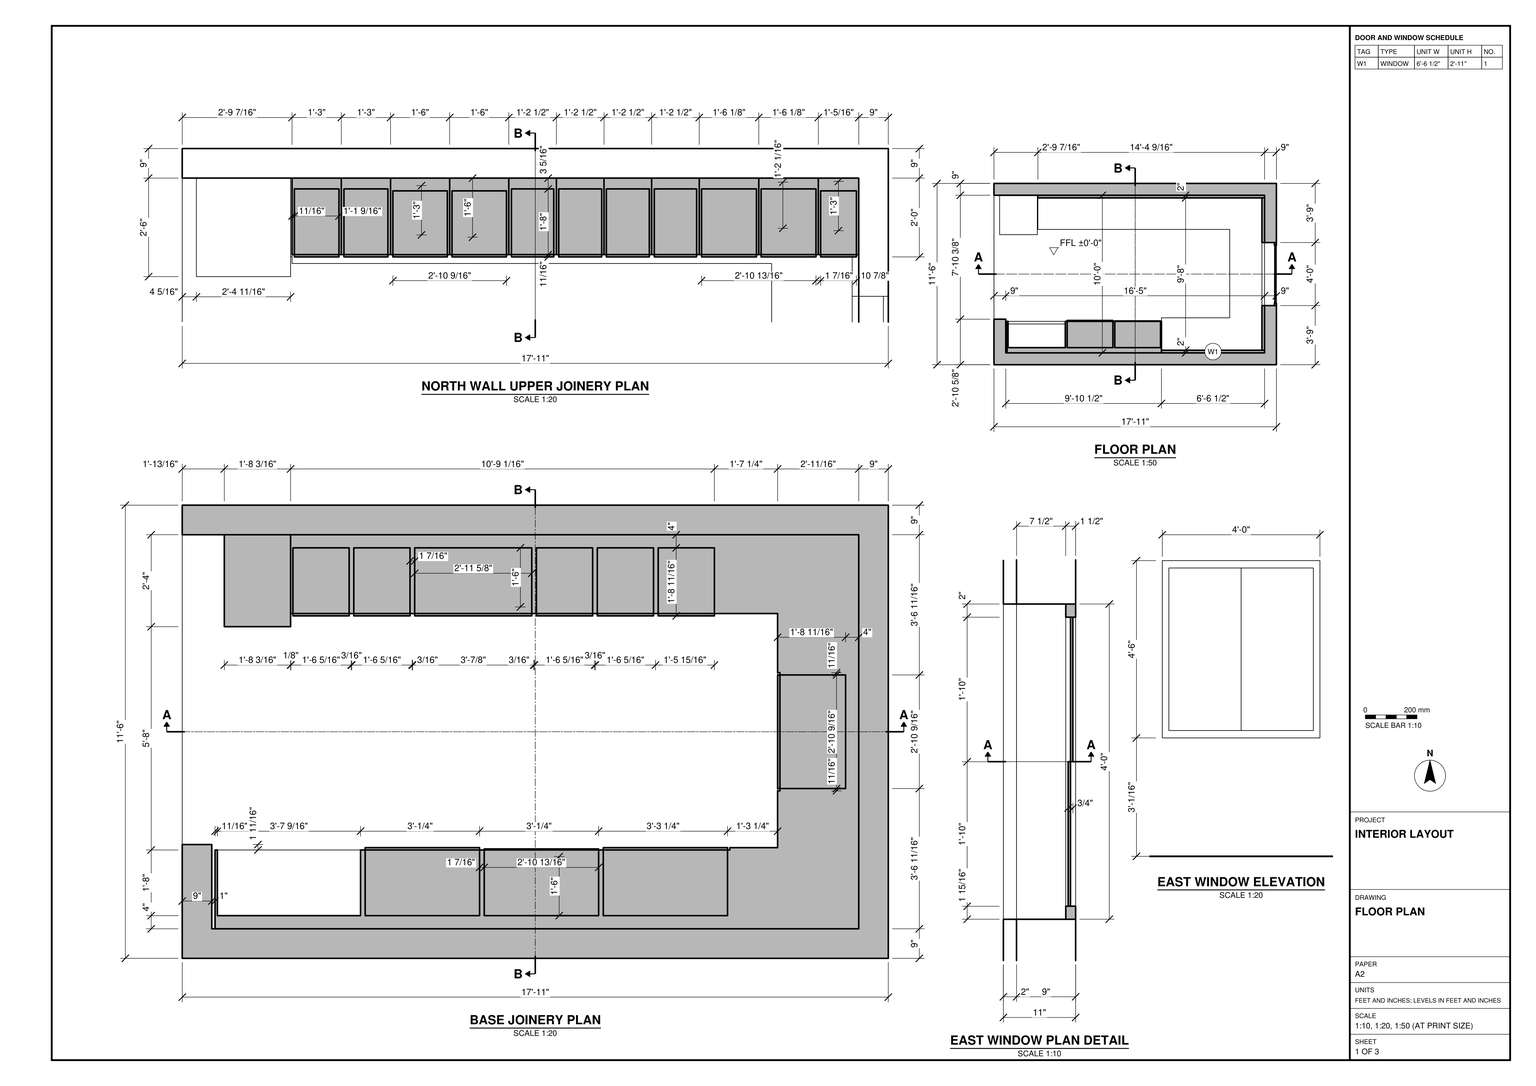
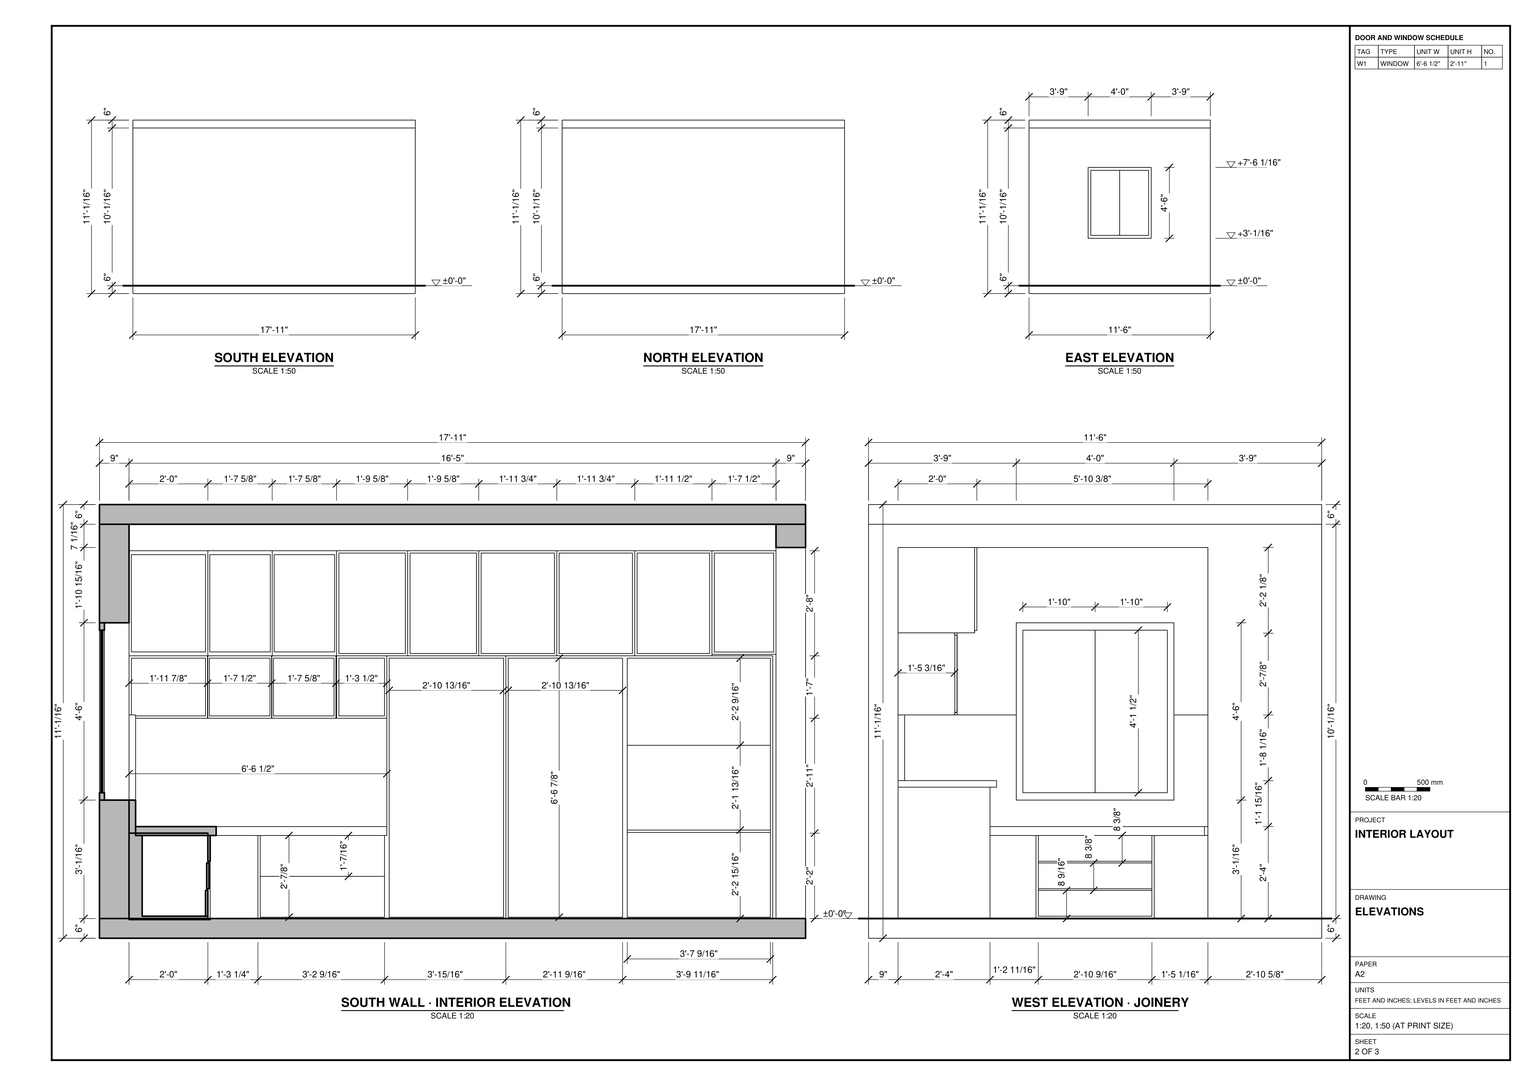
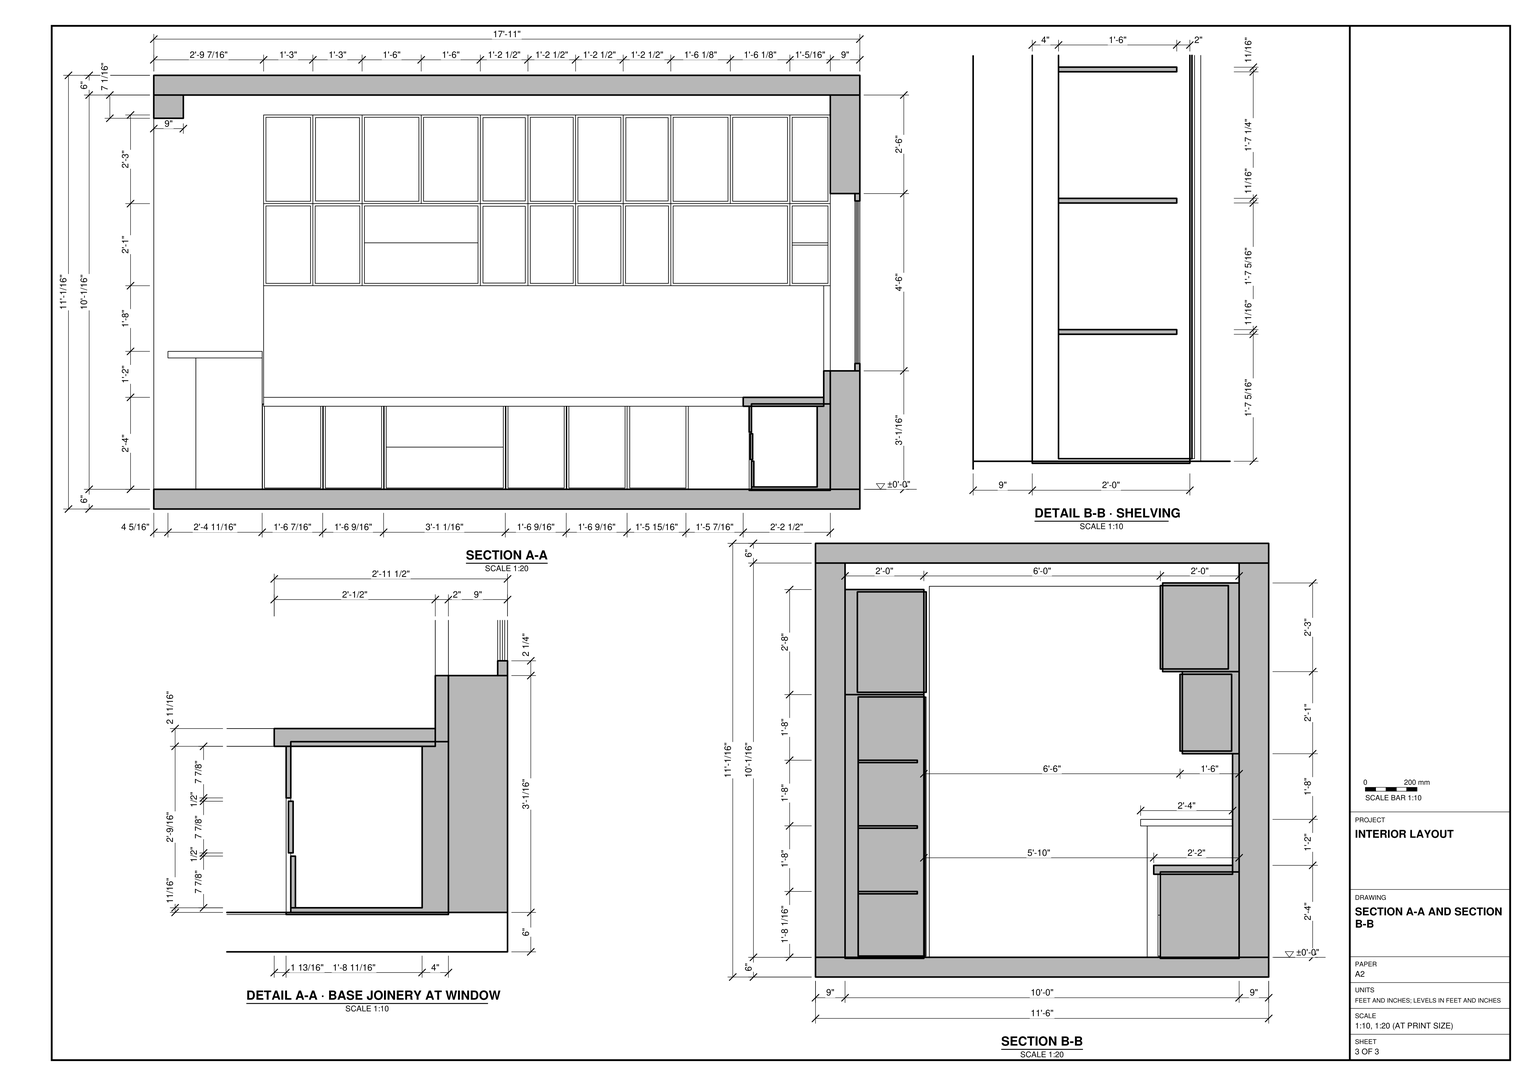
Build the room and its fitted joinery in SketchUp using task_files/diagram_01.pdf. Work in feet and inches. Set the finished floor level to ±0'-0". The overall shell measures 17'-11" east to west, 11'-6" north to south and 11'-1/16" high. Model the floor slab, top slab and walls at the thicknesses drawn, retaining the open portion of the west side shown in plan. Place the windows from the floor plan and use the east window detail for its frame and central division.

Use the base joinery plan to lay out the cabinets along the north and south walls and the connecting run beneath the east window. On the north wall, model the counter over the base units and the two tiers of upper cabinets. Use the sections to set the different cabinet depths. On the south wall, distinguish the low counter area, the tall storage bays and the stacked compartments beneath the continuous upper row. Include the drawer divisions below the east window and the internal shelving shown in detail.

Keep shell elements and individual joinery pieces in separate groups or components, and use components for repeated parts. Any decor or loose items may be suitable library components. Save one SketchUp model as output_files/fitted_storage_room_with_perimeter_cabinetry.skp.

# SketchUp Ruby script. Lengths in inches.
U = 1.inch
M = Sketchup.active_model
def pt(a) = Geom::Point3d.new(a.map { |v| v * U })
def face(e, loops, mat)
  f = e.add_face(loops[0].map { |a| pt(a) })
  loops[1..].each { |l| e.add_face(l.map { |a| pt(a) }).erase! }
  f.material = f.back_material = mat if mat
  f
end
# faces: each face lists its corners as indices into pts; further lists are holes
def faces(e, pts, list, mat = nil) = list.each { |f| face(e, (f[0].is_a?(Array) ? f : [f]).map { |l| l.map { |i| pts[i] } }, mat) }
# xy, xz, yz: faces in a plane at the given z, y or x. An outline is a flat list of corners, or four numbers for a rectangle; further outlines are holes
def ring(l) = l.size == 4 ? [[l[0], l[1]], [l[2], l[1]], [l[2], l[3]], [l[0], l[3]]] : l.each_slice(2).to_a
def flat(e, list, mat, &to3) = list.each { |f| face(e, (f[0].is_a?(Array) ? f : [f]).map { |l| ring(l).map { |u, v| to3.(u, v) } }, mat) }
def xy(e, z, list, mat = nil) = flat(e, list, mat) { |x, y| [x, y, z] }
def xz(e, y, list, mat = nil) = flat(e, list, mat) { |x, z| [x, y, z] }
def yz(e, x, list, mat = nil) = flat(e, list, mat) { |y, z| [x, y, z] }
def lines(e, pts, list) = list.each { |a, b| e.add_line(pt(pts[a]), pt(pts[b])) }
# prism: a flat outline (further loops are holes) pulled along v
def prism(e, loops, v, mat = nil)
  f = face(e, loops, mat); d = Geom::Vector3d.new(v.map { |x| x * U })
  f.pushpull(f.normal.samedirection?(d) ? d.length : -d.length)
end
def box(e, o, s, mat = nil) = prism(e, [[o, [o[0] + s[0], o[1], o[2]], [o[0] + s[0], o[1] + s[1], o[2]], [o[0], o[1] + s[1], o[2]]]], [0, 0, s[2]], mat)
def at(x, y, z, deg = 0) = Geom::Transformation.translation(pt([x, y, z])) * Geom::Transformation.rotation(ORIGIN, Z_AXIS, deg.degrees)
def axes(o, x, y, z) = Geom::Transformation.new([*x, 0, *y, 0, *z, 0, *pt(o).to_a, 1])
def part(name) = M.definitions.add(name)
# library, detail: a bought-in or finely detailed component or shape, given as its bounding box
def library(name, o, s) = part(name).tap { |d| box(d.entities, o, s) }
def detail(e, o, s) = box(e.add_group.entities, o, s)
def put(e, d, t, mat = nil) = e.add_instance(d, t).tap { |i| i.material = mat if mat }
def group(e, t, mat = nil) = e.add_group.tap { |g| g.transformation = t; g.material = mat if mat }.entities
root = M.entities
M.materials.add("Aluminium Black Anodized Fingerprints 15cm").color = [38, 38, 38]
M.materials.add("Glass Red 001").color = [0, 0, 0]
M.materials["Glass Red 001"].alpha = 0.1
M.materials.add("Marble Black 100cm").color = [32, 32, 32]
M.materials.add("Marble White 100cm").color = [222, 222, 222]
M.materials.add("Wall Paint Fine Grain 01 Yellow 100cm").color = [207, 190, 139]
M.materials.add("wadrobe paint").color = [208, 160, 134]
M.materials["wadrobe paint"].alpha = 0.5
c1 = part("Group92\#1")
p = [[0,0,0],[0,0,-10.7],[-3.66,0,-10.7],[23.84,-10.79,0],[-23.84,-10.79,0],[23.84,10.79,0],
  [23.84,0,0],[-23.84,10.79,0],[3.66,0,-10.7],[-23.84,0,0],[0,0,-17.31]]
lines(c1.entities,p,[[0,1],[1,2],[3,4],[5,6],[7,5],[1,8],[9,0],[0,6],[8,10],[4,9],[6,3],[2,10],
  [9,7]])
c2 = part("Rectangle Light")
put(c2.entities,c1,at(0,0,0))
c3 = part("Group\#13")
box(c3.entities,[0,0,0],[22.58,17.58,0.71])
c4 = part("Group\#14")
xy(c4.entities,0,[[0,0,24,19]])
xy(c4.entities,2,[[0.71,0.71,23.29,18.29]])
xy(c4.entities,18,[[[0,0,24,19],[0.71,0.71,23.29,18.29]]])
xz(c4.entities,0,[[0,0,24,18]])
xz(c4.entities,0.71,[[0.71,2,23.29,18]])
xz(c4.entities,18.29,[[0.71,2,23.29,18]])
xz(c4.entities,19,[[0,0,24,18]])
yz(c4.entities,0,[[0,0,19,18]])
yz(c4.entities,0.71,[[0.71,2,18.29,18]])
yz(c4.entities,23.29,[[0.71,2,18.29,18]])
yz(c4.entities,24,[[0,0,19,18]])
put(c4.entities,c3,at(0.71,0.71,18))
c5 = part("Group\#50")
xy(c5.entities,0,[[0,-17.29,15,0]])
xy(c5.entities,0.71,[[0.71,-17.29,14.29,-2.29]])
xy(c5.entities,24.29,[[0.71,-17.29,14.29,-2.29]])
xy(c5.entities,25,[[0,-17.29,15,0]])
xz(c5.entities,-17.29,[[[0,0,15,25],[0.71,0.71,14.29,24.29]]])
xz(c5.entities,-2.29,[[0.71,0.71,14.29,24.29]])
xz(c5.entities,0,[[0,0,15,25]])
yz(c5.entities,0,[[-17.29,0,0,25]])
yz(c5.entities,0.71,[[-17.29,0.71,-2.29,24.29]])
yz(c5.entities,14.29,[[-17.29,0.71,-2.29,24.29]])
yz(c5.entities,15,[[-17.29,0,0,25]])
g1 = group(c5.entities,at(0.71,-17.29,0.71))
box(g1,[0,-0.71,0],[13.58,0.71,23.58])
c6 = part("Group\#64")
xy(c6.entities,0,[[0,-24,18,0]])
xy(c6.entities,0.71,[[0.71,-24,17.29,-4]])
xy(c6.entities,26.29,[[0.71,-24,17.29,-4]])
xy(c6.entities,27,[[0,-24,18,0]])
xz(c6.entities,-24,[[[0,0,18,27],[0.71,0.71,17.29,26.29]]])
xz(c6.entities,-4,[[0.71,0.71,17.29,26.29]])
xz(c6.entities,0,[[0,0,18,27]])
yz(c6.entities,0,[[-24,0,0,27]])
yz(c6.entities,0.71,[[-24,0.71,-4,26.29]])
yz(c6.entities,17.29,[[-24,0.71,-4,26.29]])
yz(c6.entities,18,[[-24,0,0,27]])
g2 = group(c6.entities,at(0.71,-24,0.71))
box(g2,[0,-0.71,0],[16.58,0.71,25.58])
c7 = part("Group\#3")
box(c7.entities,[0,0,0],[37.83,0.71,12.45])
c8 = part("Group\#4")
box(c8.entities,[-0.71,0,0],[0.71,34.58,7.86])
c9 = part("Group\#6")
box(c9.entities,[0,0,-0.35],[34.83,18,0.7])
c10 = part("Group\#8")
box(c10.entities,[0,0,-0.35],[43.58,18,0.7])
put(root,c2,axes([105.16,70.09,120.0625],[2.9512,0,0],[0,-1.82,0],[0,0,1.00058]))
g3 = group(root,at(9,9,0))
xy(g3,0,[[-9,-9,-9,25.65,0,25.65,0,0,197,0,197,120,-9,120,-9,129,206,129,206,-9]])
xy(g3,0,[[0,0,197,0,197,120,-9,120,-9,25.65,0,25.65]],"Marble Black 100cm")
xy(g3,36.0625,[[197,36,206,84]])
xy(g3,90.0625,[[197,36,206,84]])
xy(g3,112.98,[[-9,25.65,0,120]])
xy(g3,120.0625,[[[-9,-9,206,129],[0,0,197,120]]])
xz(g3,-9,[[-9,0,206,120.0625]])
xz(g3,0,[[118.5,61,118.5,80,19.5,80,19.5,80.45,0,80.45,0,112,133.8,112,133.8,61]])
xz(g3,0,[[0,0,0,80.45,19.5,80.45,19.5,80,118.5,80,118.5,61,133.8,61,133.8,112,0,112,0,120.0625,197,120.0625,197,0]],"Wall Paint Fine Grain 01 Yellow 100cm")
xz(g3,25.65,[[-9,0,0,112.98]])
xz(g3,36,[[197,36.0625,206,90.0625]])
xz(g3,84,[[197,36.0625,206,90.0625]])
xz(g3,120,[[3.8125,-0.3125,24,0],[3.8125,0,24,40],[24.4375,62,54.4375,62,54.4375,87,90.4375,87,90.4375,62,184.6875,62,184.6875,87,197,87,197,114,24.4375,114]])
xz(g3,120,[[-9,0,3.8125,0,3.8125,40,24,40,24,0,197,0,197,87,184.6875,87,184.6875,62,90.4375,62,90.4375,87,54.4375,87,54.4375,62,24.4375,62,24.4375,114,197,114,197,120.0625,0,120.0625,0,112.98,-9,112.98]],"Wall Paint Fine Grain 01 Yellow 100cm")
xz(g3,129,[[-9,0,206,120.0625]])
yz(g3,-9,[[-9,0,-9,120.0625,129,120.0625,129,0,120,0,120,112.98,25.65,112.98,25.65,0]])
yz(g3,0,[[0,0,25.65,0,25.65,112.98,120,112.98,120,120.0625,0,120.0625]])
yz(g3,197,[[[0,0,120,120.0625],[2,26,118,26,118,62,84,62,84,90.0625,36,90.0625,36,62,2,62]]],"Wall Paint Fine Grain 01 Yellow 100cm")
yz(g3,206,[[[-9,0,129,120.0625],[36,36.0625,84,90.0625]]])
g4 = group(g3,at(197,0,26),"Marble Black 100cm")
box(g4,[-78.5,0,0],[78.5,2,35],"Marble Black 100cm")
g5 = group(g3,at(197,0,80))
xz(g5,0,[[-24,0,0,32]])
put(g3,c4,axes([197,0,61],[-1,0,0],[0,0,1],[0,1,0]),"wadrobe paint")
g6 = group(g3,at(197,0,80),"wadrobe paint")
xy(g6,0,[[-24,0,0,18]])
xy(g6,1.19,[[-23.29,2,-0.71,18]])
xy(g6,30.81,[[-23.29,2,-0.71,18]])
xy(g6,32,[[-24,0,0,18]])
xz(g6,0,[[-24,0,0,32]])
xz(g6,2,[[-23.29,1.19,-0.71,30.81]])
xz(g6,18,[[[-24,0,0,32],[-23.29,1.19,-0.71,30.81]]])
yz(g6,-24,[[0,0,18,32]])
yz(g6,-23.29,[[2,1.19,18,30.81]])
yz(g6,-0.71,[[2,1.19,18,30.81]])
yz(g6,0,[[0,0,18,32]])
put(g6,c3,axes([-0.71,18,1.19],[-1,0,0],[0,0,1.68421],[0,1,0]))
put(g3,c4,axes([173.1,0,61],[-0.8166,0,0],[0,0,1],[0,1,0]),"wadrobe paint")
put(g3,c4,axes([173,0,80],[-0.8166,0,0],[0,0,1.68421],[0,1,0]),"wadrobe paint")
put(g3,c4,axes([153.6,0,61],[-0.8166,0,0],[0,0,1],[0,1,0]),"wadrobe paint")
put(g3,c4,axes([153.4,0,80],[-0.8166,0,0],[0,0,1.68421],[0,1,0]),"wadrobe paint")
g7 = group(g3,at(118.5,0,61),"wadrobe paint")
xy(g7,0,[[0,0,15.3,18]])
xy(g7,0.71,[[0.71,2,14.59,18]])
xy(g7,18.29,[[0.71,2,14.59,18]])
xy(g7,19,[[0,0,15.3,18]])
xz(g7,0,[[0,0,15.3,19]])
xz(g7,2,[[0.71,0.71,14.59,18.29]])
xz(g7,18,[[[0,0,15.3,19],[0.71,0.71,14.59,18.29]]])
yz(g7,0,[[0,0,18,19]])
yz(g7,0.71,[[2,0.71,18,18.29]])
yz(g7,14.59,[[2,0.71,18,18.29]])
yz(g7,15.3,[[0,0,18,19]])
g8 = group(g7,at(0.71,18,0.71))
box(g8,[0,0,0],[13.89,0.71,17.58])
g9 = group(g3,at(112.15,0,80),"wadrobe paint")
xy(g9,0,[[0,0,21.65,18]])
xy(g9,0.71,[[0.71,2,20.94,18]])
xy(g9,31.29,[[0.71,2,20.94,18]])
xy(g9,32,[[0,0,21.65,18]])
xz(g9,0,[[0,0,21.65,32]])
xz(g9,2,[[0.71,0.71,20.94,31.29]])
xz(g9,18,[[[0,0,21.65,32],[0.71,0.71,20.94,31.29]]])
yz(g9,0,[[0,0,18,32]])
yz(g9,0.71,[[2,0.71,18,31.29]])
yz(g9,20.94,[[2,0.71,18,31.29]])
yz(g9,21.65,[[0,0,18,32]])
g10 = group(g9,at(0.71,18,0.71))
box(g10,[0,0,0],[20.23,0.71,30.58])
g11 = group(g3,at(90.5,0,80),"wadrobe paint")
xy(g11,0,[[0,0,21.65,24]])
xy(g11,0.71,[[0.71,3.75,20.94,24]])
xy(g11,31.29,[[0.71,3.75,20.94,24]])
xy(g11,32,[[0,0,21.65,24]])
xz(g11,0,[[0,0,21.65,32]])
xz(g11,3.75,[[0.71,0.71,20.94,31.29]])
xz(g11,24,[[[0,0,21.65,32],[0.71,0.71,20.94,31.29]]])
yz(g11,0,[[0,0,24,32]])
yz(g11,0.71,[[3.75,0.71,24,31.29]])
yz(g11,20.94,[[3.75,0.71,24,31.29]])
yz(g11,21.65,[[0,0,24,32]])
g12 = group(g11,at(0.71,24,0.71))
box(g12,[0,0,0],[20.23,0.71,30.58])
g13 = group(g3,at(66.75,0,80),"wadrobe paint")
xy(g13,0,[[0,0,23.75,24]])
xy(g13,0.71,[[0.71,3.8125,23.04,24]])
xy(g13,31.29,[[0.71,3.8125,23.04,24]])
xy(g13,32,[[0,0,23.75,24]])
xz(g13,0,[[0,0,23.75,32]])
xz(g13,3.8125,[[0.71,0.71,23.04,31.29]])
xz(g13,24,[[[0,0,23.75,32],[0.71,0.71,23.04,31.29]]])
yz(g13,0,[[0,0,24,32]])
yz(g13,0.71,[[3.8125,0.71,24,31.29]])
yz(g13,23.04,[[3.8125,0.71,24,31.29]])
yz(g13,23.75,[[0,0,24,32]])
g14 = group(g13,at(0.71,24,0.71))
box(g14,[0,0,0],[22.33,0.71,30.58])
g15 = group(g3,at(43,0,80),"wadrobe paint")
xy(g15,0,[[0,0,23.75,24]])
xy(g15,0.71,[[0.71,4,23.04,24]])
xy(g15,31.29,[[0.71,4,23.04,24]])
xy(g15,32,[[0,0,23.75,24]])
xz(g15,0,[[0,0,23.75,32]])
xz(g15,4,[[0.71,0.71,23.04,31.29]])
xz(g15,24,[[[0,0,23.75,32],[0.71,0.71,23.04,31.29]]])
yz(g15,0,[[0,0,24,32]])
yz(g15,0.71,[[4,0.71,24,31.29]])
yz(g15,23.04,[[4,0.71,24,31.29]])
yz(g15,23.75,[[0,0,24,32]])
g16 = group(g15,at(0.71,24,0.71))
box(g16,[0,0,0],[22.33,0.71,30.58])
g17 = group(g3,at(19.5,0,80),"wadrobe paint")
xy(g17,0,[[0,0,23.5,24]])
xy(g17,0.71,[[0.71,4,22.79,24]])
xy(g17,31.29,[[0.71,4,22.79,24]])
xy(g17,32,[[0,0,23.5,24]])
xz(g17,0,[[0,0,23.5,32]])
xz(g17,4,[[0.71,0.71,22.79,31.29]])
xz(g17,24,[[[0,0,23.5,32],[0.71,0.71,22.79,31.29]]])
yz(g17,0,[[0,0,24,32]])
yz(g17,0.71,[[4,0.71,24,31.29]])
yz(g17,22.79,[[4,0.71,24,31.29]])
yz(g17,23.5,[[0,0,24,32]])
g18 = group(g17,at(0.71,24,0.71))
box(g18,[0,0,0],[22.08,0.71,30.58])
g19 = group(g3,at(0,0,80.45),"wadrobe paint")
xy(g19,0,[[0,0,19.5,24]])
xy(g19,0.71,[[0.71,4,18.79,24]])
xy(g19,30.84,[[0.71,4,18.79,24]])
xy(g19,31.55,[[0,0,19.5,24]])
xz(g19,0,[[0,0,19.5,31.55]])
xz(g19,4,[[0.71,0.71,18.79,30.84]])
xz(g19,24,[[[0,0,19.5,31.55],[0.71,0.71,18.79,30.84]]])
yz(g19,0,[[0,0,24,31.55]])
yz(g19,0.71,[[4,0.71,24,30.84]])
yz(g19,18.79,[[4,0.71,24,30.84]])
yz(g19,19.5,[[0,0,24,31.55]])
g20 = group(g19,at(0.71,24,0.71))
box(g20,[0,0,0],[18.08,0.71,30.13])
g21 = group(g3,at(184.6875,120,87),"wadrobe paint")
xy(g21,0,[[0,-23.3125,12.3125,0]])
xy(g21,0.71,[[0.71,-23.3125,11.6,-3.89]])
xy(g21,26.29,[[0.71,-23.3125,11.6,-3.89]])
xy(g21,27,[[0,-23.3125,12.3125,0]])
xz(g21,-23.3125,[[[0,0,12.3125,27],[0.71,0.71,11.6,26.29]]])
xz(g21,-3.89,[[0.71,0.71,11.6,26.29]])
xz(g21,0,[[0,0,12.3125,27]])
yz(g21,0,[[-23.3125,0,0,27]])
yz(g21,0.71,[[-23.3125,0.71,-3.89,26.29]])
yz(g21,11.6,[[-23.3125,0.71,-3.89,26.29]])
yz(g21,12.3125,[[-23.3125,0,0,27]])
g22 = group(g21,at(0.71,-23.3125,0.71))
box(g22,[0,-0.6875,0],[10.9,0.6875,25.58])
g23 = group(g3,at(148.4375,120,62),"wadrobe paint")
xy(g23,0,[[0,-17.29,36.25,0]])
xy(g23,0.71,[[0.71,-17.29,35.54,-1.23]])
xy(g23,24.29,[[0.71,-17.29,35.54,-1.23]])
xy(g23,25,[[0,-17.29,36.25,0]])
xz(g23,-17.29,[[[0,0,36.25,25],[0.71,0.71,35.54,24.29]]],"Aluminium Black Anodized Fingerprints 15cm")
xz(g23,-1.23,[[0.71,0.71,35.54,24.29]])
xz(g23,0,[[0,0,36.25,25]])
yz(g23,0,[[-17.29,0,0,25]])
yz(g23,0.71,[[-17.29,0.71,-1.23,24.29]])
yz(g23,35.54,[[-17.29,0.71,-1.23,24.29]])
yz(g23,36.25,[[-17.29,0,0,25]])
g24 = group(g23,at(0.71,-17.29,12.71))
box(g24,[0,2,-0.35],[34.83,14.0625,0.7])
g25 = group(g23,at(0.71,-17.29,0.71),"Glass Red 001")
box(g25,[0,-0.71,0],[34.83,0.71,23.58])
g26 = group(g3,at(54.4375,120,62),"wadrobe paint")
xy(g26,0,[[0,-17.29,36,0]])
xy(g26,0.71,[[0.71,-17.29,35.29,-2.29]])
xy(g26,24.29,[[0.71,-17.29,35.29,-2.29]])
xy(g26,25,[[0,-17.29,36,0]])
xz(g26,-17.29,[[[0,0,36,25],[0.71,0.71,35.29,24.29]]])
xz(g26,-2.29,[[0.71,0.71,35.29,24.29]])
xz(g26,0,[[0,0,36,25]])
yz(g26,0,[[-17.29,0,0,25]])
yz(g26,0.71,[[-17.29,0.71,-2.29,24.29]])
yz(g26,35.29,[[-17.29,0.71,-2.29,24.29]])
yz(g26,36,[[-17.29,0,0,25]])
g27 = group(g26,at(0.71,-2.29,12.71))
box(g27,[0,-15,-0.35],[34.58,15,0.7])
g28 = group(g26,at(0.71,-17.29,13.0625))
box(g28,[0,-0.71,0],[34.58,0.71,11.23])
g29 = group(g26,at(0.71,-17.29,0.71))
box(g29,[0,-0.71,0],[34.58,0.71,12.35])
g30 = group(g3,at(133.9375,120,62),"wadrobe paint")
xy(g30,0,[[0,-17.29,14.5,0]])
xy(g30,0.71,[[0.71,-17.29,13.79,-2.23]])
xy(g30,24.29,[[0.71,-17.29,13.79,-2.23]])
xy(g30,25,[[0,-17.29,14.5,0]])
xz(g30,-17.29,[[[0,0,14.5,25],[0.71,0.71,13.79,24.29]]])
xz(g30,-2.23,[[0.71,0.71,13.79,24.29]])
xz(g30,0,[[0,0,14.5,25]])
yz(g30,0,[[-17.29,0,0,25]])
yz(g30,0.71,[[-17.29,0.71,-2.23,24.29]])
yz(g30,13.79,[[-17.29,0.71,-2.23,24.29]])
yz(g30,14.5,[[-17.29,0,0,25]])
g31 = group(g30,at(0.71,-17.29,0.71))
box(g31,[0,-0.71,0],[13.08,0.71,23.58])
g32 = group(g3,at(119.4375,120,62),"wadrobe paint")
xy(g32,0,[[0,-17.23,14.5,0]])
xy(g32,0.71,[[0.71,-17.23,13.79,-2.23]])
xy(g32,24.29,[[0.71,-17.23,13.79,-2.23]])
xy(g32,25,[[0,-17.23,14.5,0]])
xz(g32,-17.23,[[[0,0,14.5,25],[0.71,0.71,13.79,24.29]]])
xz(g32,-2.23,[[0.71,0.71,13.79,24.29]])
xz(g32,0,[[0,0,14.5,25]])
yz(g32,0,[[-17.23,0,0,25]])
yz(g32,0.71,[[-17.23,0.71,-2.23,24.29]])
yz(g32,13.79,[[-17.23,0.71,-2.23,24.29]])
yz(g32,14.5,[[-17.23,0,0,25]])
g33 = group(g32,at(0.71,-17.23,0.71))
box(g33,[0,-0.71,0],[13.08,0.71,23.58])
g34 = group(g3,at(104.9375,120,62),"wadrobe paint")
xy(g34,0,[[0,-17.29,14.5,0]])
xy(g34,0.71,[[0.71,-17.29,13.79,-2.29]])
xy(g34,24.29,[[0.71,-17.29,13.79,-2.29]])
xy(g34,25,[[0,-17.29,14.5,0]])
xz(g34,-17.29,[[[0,0,14.5,25],[0.71,0.71,13.79,24.29]]])
xz(g34,-2.29,[[0.71,0.71,13.79,24.29]])
xz(g34,0,[[0,0,14.5,25]])
yz(g34,0,[[-17.29,0,0,25]])
yz(g34,0.71,[[-17.29,0.71,-2.29,24.29]])
yz(g34,13.79,[[-17.29,0.71,-2.29,24.29]])
yz(g34,14.5,[[-17.29,0,0,25]])
g35 = group(g34,at(0.71,-17.29,0.71))
box(g35,[0,-0.71,0],[13.08,0.71,23.58])
g36 = group(g3,at(90.4375,120,62),"wadrobe paint")
xy(g36,0,[[0,-17.29,14.5,0]])
xy(g36,0.81,[[0.81,-17.29,13.69,-2.29]])
xy(g36,24.19,[[0.81,-17.29,13.69,-2.29]])
xy(g36,25,[[0,-17.29,14.5,0]])
xz(g36,-17.29,[[[0,0,14.5,25],[0.81,0.81,13.69,24.19]]])
xz(g36,-2.29,[[0.81,0.81,13.69,24.19]])
xz(g36,0,[[0,0,14.5,25]])
yz(g36,0,[[-17.29,0,0,25]])
yz(g36,0.81,[[-17.29,0.81,-2.29,24.19]])
yz(g36,13.69,[[-17.29,0.81,-2.29,24.19]])
yz(g36,14.5,[[-17.29,0,0,25]])
g37 = group(g36,at(0.81,-17.29,0.81))
box(g37,[0,-0.71,0],[12.89,0.71,23.39])
put(g3,c5,at(24.4375,120,62),"wadrobe paint")
put(g3,c5,at(39.4375,120,62),"wadrobe paint")
g38 = group(g3,at(166.5625,120,87),"wadrobe paint")
xy(g38,0,[[0,-23.29,18.125,0]])
xy(g38,0.71,[[0.71,-23.29,17.42,-3.29]])
xy(g38,26.29,[[0.71,-23.29,17.42,-3.29]])
xy(g38,27,[[0,-23.29,18.125,0]])
xz(g38,-23.29,[[[0,0,18.125,27],[0.71,0.71,17.42,26.29]]])
xz(g38,-3.29,[[0.71,0.71,17.42,26.29]])
xz(g38,0,[[0,0,18.125,27]])
yz(g38,0,[[-23.29,0,0,27]])
yz(g38,0.71,[[-23.29,0.71,-3.29,26.29]])
yz(g38,17.42,[[-23.29,0.71,-3.29,26.29]])
yz(g38,18.125,[[-23.29,0,0,27]])
g39 = group(g38,at(0.71,-23.29,0.71))
box(g39,[0,-0.71,0],[16.71,0.71,25.58])
g40 = group(g3,at(148.4375,120,87),"wadrobe paint")
xy(g40,0,[[0,-23.29,18.125,0]])
xy(g40,0.71,[[0.71,-23.29,17.42,-3.29]])
xy(g40,26.29,[[0.71,-23.29,17.42,-3.29]])
xy(g40,27,[[0,-23.29,18.125,0]])
xz(g40,-23.29,[[[0,0,18.125,27],[0.71,0.71,17.42,26.29]]])
xz(g40,-3.29,[[0.71,0.71,17.42,26.29]])
xz(g40,0,[[0,0,18.125,27]])
yz(g40,0,[[-23.29,0,0,27]])
yz(g40,0.71,[[-23.29,0.71,-3.29,26.29]])
yz(g40,17.42,[[-23.29,0.71,-3.29,26.29]])
yz(g40,18.125,[[-23.29,0,0,27]])
g41 = group(g40,at(0.71,-23.29,0.71))
box(g41,[0,-0.71,0],[16.71,0.71,25.58])
g42 = group(g3,at(133.9375,120,87),"wadrobe paint")
xy(g42,0,[[0,-23.29,14.5,0]])
xy(g42,0.81,[[0.81,-23.29,13.69,-3.29]])
xy(g42,26.19,[[0.81,-23.29,13.69,-3.29]])
xy(g42,27,[[0,-23.29,14.5,0]])
xz(g42,-23.29,[[[0,0,14.5,27],[0.81,0.81,13.69,26.19]]])
xz(g42,-3.29,[[0.81,0.81,13.69,26.19]])
xz(g42,0,[[0,0,14.5,27]])
yz(g42,0,[[-23.29,0,0,27]])
yz(g42,0.81,[[-23.29,0.81,-3.29,26.19]])
yz(g42,13.69,[[-23.29,0.81,-3.29,26.19]])
yz(g42,14.5,[[-23.29,0,0,27]])
g43 = group(g42,at(0.81,-23.29,0.81))
box(g43,[0,-0.71,0],[12.89,0.71,25.39])
g44 = group(g3,at(119.4375,120,87),"wadrobe paint")
xy(g44,0,[[0,-23.29,14.5,0]])
xy(g44,0.71,[[0.71,-23.29,13.79,-3.29]])
xy(g44,26.29,[[0.71,-23.29,13.79,-3.29]])
xy(g44,27,[[0,-23.29,14.5,0]])
xz(g44,-23.29,[[[0,0,14.5,27],[0.71,0.71,13.79,26.29]]])
xz(g44,-3.29,[[0.71,0.71,13.79,26.29]])
xz(g44,0,[[0,0,14.5,27]])
yz(g44,0,[[-23.29,0,0,27]])
yz(g44,0.71,[[-23.29,0.71,-3.29,26.29]])
yz(g44,13.79,[[-23.29,0.71,-3.29,26.29]])
yz(g44,14.5,[[-23.29,0,0,27]])
g45 = group(g44,at(0.71,-23.29,0.71))
box(g45,[0,-0.71,0],[13.08,0.71,25.58])
g46 = group(g3,at(104.9375,120,87),"wadrobe paint")
xy(g46,0,[[0,-23.29,14.5,0]])
xy(g46,0.71,[[0.71,-23.29,13.79,-3.29]])
xy(g46,26.29,[[0.71,-23.29,13.79,-3.29]])
xy(g46,27,[[0,-23.29,14.5,0]])
xz(g46,-23.29,[[[0,0,14.5,27],[0.71,0.71,13.79,26.29]]])
xz(g46,-3.29,[[0.71,0.71,13.79,26.29]])
xz(g46,0,[[0,0,14.5,27]])
yz(g46,0,[[-23.29,0,0,27]])
yz(g46,0.71,[[-23.29,0.71,-3.29,26.29]])
yz(g46,13.79,[[-23.29,0.71,-3.29,26.29]])
yz(g46,14.5,[[-23.29,0,0,27]])
g47 = group(g46,at(0.71,-23.29,0.71))
box(g47,[0,-0.71,0],[13.08,0.71,25.58])
g48 = group(g3,at(90.4375,120,87),"wadrobe paint")
xy(g48,0,[[0,-23.29,14.5,0]])
xy(g48,0.81,[[0.81,-23.29,13.69,-3.29]])
xy(g48,26.19,[[0.81,-23.29,13.69,-3.29]])
xy(g48,27,[[0,-23.29,14.5,0]])
xz(g48,-23.29,[[[0,0,14.5,27],[0.81,0.81,13.69,26.19]]])
xz(g48,-3.29,[[0.81,0.81,13.69,26.19]])
xz(g48,0,[[0,0,14.5,27]])
yz(g48,0,[[-23.29,0,0,27]])
yz(g48,0.81,[[-23.29,0.81,-3.29,26.19]])
yz(g48,13.69,[[-23.29,0.81,-3.29,26.19]])
yz(g48,14.5,[[-23.29,0,0,27]])
g49 = group(g48,at(0.81,-23.29,0.81))
box(g49,[0,-0.71,0],[12.89,0.71,25.39])
put(g3,c6,axes([72.4375,120,87],[1,0,0],[0,0.97132,0],[0,0,1]),"wadrobe paint")
put(g3,c6,axes([54.4375,120,87],[1,0,0],[0,0.97132,0],[0,0,1]),"wadrobe paint")
g50 = group(g3,at(39.4375,120,87),"wadrobe paint")
xy(g50,0,[[0,-23.29,15,0]])
xy(g50,0.81,[[0.81,-23.29,14.19,-3.29]])
xy(g50,26.19,[[0.81,-23.29,14.19,-3.29]])
xy(g50,27,[[0,-23.29,15,0]])
xz(g50,-23.29,[[[0,0,15,27],[0.81,0.81,14.19,26.19]]])
xz(g50,-3.29,[[0.81,0.81,14.19,26.19]])
xz(g50,0,[[0,0,15,27]])
yz(g50,0,[[-23.29,0,0,27]])
yz(g50,0.81,[[-23.29,0.81,-3.29,26.19]])
yz(g50,14.19,[[-23.29,0.81,-3.29,26.19]])
yz(g50,15,[[-23.29,0,0,27]])
g51 = group(g50,at(0.81,-23.29,0.81))
box(g51,[0,-0.71,0],[13.39,0.71,25.39])
g52 = group(g3,at(24.4375,120,87),"wadrobe paint")
xy(g52,0,[[0,-23.29,15,0]])
xy(g52,0.71,[[0.71,-23.29,14.29,-3.29]])
xy(g52,26.29,[[0.71,-23.29,14.29,-3.29]])
xy(g52,27,[[0,-23.29,15,0]])
xz(g52,-23.29,[[[0,0,15,27],[0.71,0.71,14.29,26.29]]])
xz(g52,-3.29,[[0.71,0.71,14.29,26.29]])
xz(g52,0,[[0,0,15,27]])
yz(g52,0,[[-23.29,0,0,27]])
yz(g52,0.71,[[-23.29,0.71,-3.29,26.29]])
yz(g52,14.29,[[-23.29,0.71,-3.29,26.29]])
yz(g52,15,[[-23.29,0,0,27]])
g53 = group(g52,at(0.71,-23.29,0.71))
box(g53,[0,-0.71,0],[13.58,0.71,25.58])
g54 = group(g3,at(197,2,26),"Marble Black 100cm")
prism(g54,[[[0,82,36],[0,82,10.0625],[0,34,10.0625],[0,34,36],[0,0,36],[0,0,0],[0,116,0],[0,116,36]]],[-2,0,0],"Marble Black 100cm")
g55 = group(g3,at(3.8125,120,0),"wadrobe paint")
box(g55,[0,-28,0],[20.1875,28,40])
g56 = group(g3,at(3.8125,92,40),"Marble White 100cm")
box(g56,[-8.5,-2,0],[28.6875,30,2],"Marble White 100cm")
g57 = group(root,at(182,33,0))
xy(g57,-0.3125,[[-172,-24,-172,0,-15.25,0,-15.25,0.71,-0.71,0.71,-0.71,72,-149,72,-149,96,24,96,24,-24]])
xy(g57,0,[[-0.71,18,0,54]])
xy(g57,0.4,[[-126.29,-20,-91.46,0],[-90.04,-20,-55.21,0],[-53.79,-20,-15.96,0],[-37.07,72,-19.95,92]])
xy(g57,0.4,[[-171.29,-20,-127.71,0]],"wadrobe paint")
xy(g57,0.71,[[0,18.71,20,53.29]])
xy(g57,25.29,[[-53.79,-20,-15.96,0],[0,18.71,20,53.29],[-37.07,72,-19.95,92]])
xy(g57,26,[[-54.5,-24,24,-24,24,96,-149,96,-149,72,-0.71,72,-0.71,54,0,54,0,18,-0.71,18,-0.71,0.71,-15.25,0.71,-15.25,0,-54.5,0]])
xy(g57,79.29,[[-171.29,-20,-127.71,0],[-126.29,-20,-91.46,0],[-90.04,-20,-55.21,0]])
xy(g57,80,[[-172,-24,-54.5,0]])
xz(g57,-24,[[-172,-0.3125,24,-0.3125,24,26,-54.5,26,-54.5,80,-172,80]])
xz(g57,-20,[[-126.29,0.4,-91.46,79.29],[-90.04,0.4,-55.21,79.29],[-53.79,0.4,-15.96,25.29]])
xz(g57,-20,[[-171.29,0.4,-127.71,79.29]],"wadrobe paint")
xz(g57,0,[[[-90.75,-0.3125,-90.75,80,-54.5,80,-54.5,26,-15.25,26,-15.25,-0.3125],[-90.04,0.4,-55.21,79.29],[-53.79,0.4,-15.96,25.29]]])
xz(g57,0,[[[-172,-0.3125,-90.75,80],[-171.29,0.4,-127.71,79.29],[-126.29,0.4,-91.46,79.29]]],"wadrobe paint")
xz(g57,0.71,[[-15.25,-0.3125,-0.71,26]],"wadrobe paint")
xz(g57,18,[[-0.71,0,0,26]])
xz(g57,18.71,[[0,0.71,20,25.29]])
xz(g57,53.29,[[0,0.71,20,25.29]])
xz(g57,54,[[-0.71,0,0,26]])
xz(g57,72,[[[-149,-0.3125,-19.25,26],[-37.07,0.4,-19.95,25.29]]])
xz(g57,72,[[-19.25,-0.3125,-0.71,26]],"wadrobe paint")
xz(g57,92,[[-37.07,0.4,-19.95,25.29]])
xz(g57,96,[[-149,-0.3125,24,26]])
yz(g57,-172,[[-24,-0.3125,0,80]])
yz(g57,-171.29,[[-20,0.4,0,79.29]],"wadrobe paint")
yz(g57,-149,[[72,-0.3125,96,26]])
yz(g57,-127.71,[[-20,0.4,0,79.29]],"wadrobe paint")
yz(g57,-126.29,[[-20,0.4,0,79.29]])
yz(g57,-91.46,[[-20,0.4,0,79.29]])
yz(g57,-90.04,[[-20,0.4,0,79.29]])
yz(g57,-55.21,[[-20,0.4,0,79.29]])
yz(g57,-54.5,[[-24,26,0,80]])
yz(g57,-53.79,[[-20,0.4,0,25.29]])
yz(g57,-37.07,[[72,0.4,92,25.29]])
yz(g57,-19.95,[[72,0.4,92,25.29]])
yz(g57,-15.96,[[-20,0.4,0,25.29]])
yz(g57,-15.25,[[0,-0.3125,0.71,26]])
yz(g57,-0.71,[[0.71,-0.3125,0.71,26,18,26,18,0,54,0,54,26,72,26,72,-0.3125]],"wadrobe paint")
yz(g57,0,[[[18,0,54,26],[18.71,0.71,53.29,25.29]]])
yz(g57,20,[[18.71,0.71,53.29,25.29]])
yz(g57,24,[[-24,-0.3125,96,26]])
put(g57,c7,at(-53.79,0,12.84),"wadrobe paint")
put(g57,c7,at(-53.79,0,0.4),"wadrobe paint")
put(g57,c8,at(0,18.71,17.43),"wadrobe paint")
put(g57,c8,at(0.35,18.71,9.07),"wadrobe paint")
put(g57,c8,at(0.71,18.71,0.71),"wadrobe paint")
g58 = group(g57,at(-126.29,0,0.4),"wadrobe paint")
box(g58,[0,0,0],[34.83,0.71,78.9])
put(g57,c9,at(-90.04,-20,59.66))
put(g57,c9,at(-90.04,-20,39.68))
put(g57,c9,at(-90.04,-20,19.69))
g59 = group(g57,at(-90.04,0,0.4),"wadrobe paint")
xy(g59,0,[[0,0,34.83,0.31]])
xy(g59,78.9,[[0,0,34.83,0.31]])
xz(g59,0,[[0,0,34.83,78.9]])
xz(g59,0.31,[[0,0,34.83,78.9]],"Glass Red 001")
yz(g59,0,[[0,0,0.31,78.9]])
yz(g59,34.83,[[0,0,0.31,78.9]])
put(g57,c10,at(-171.29,-20,53.11))
put(g57,c10,at(-171.29,-20,26.58),"wadrobe paint")
g60 = group(g57,at(-171.29,0,53.88),"wadrobe paint")
box(g60,[0,0,-1.12],[43.58,0.71,26.53])
g61 = group(g57,at(-37.07,72,0.4),"wadrobe paint")
box(g61,[0,-0.71,0],[17.12,0.71,24.9])
g62 = group(g57,at(-56.32,72,-0.3125),"wadrobe paint")
xy(g62,0.71,[[0.71,0,17.83,20]])
xy(g62,25.6,[[0.71,0,17.83,20]])
xz(g62,0,[[[0.1,0.1,18.4375,26.21],[0.71,0.71,17.83,25.6]]])
xz(g62,20,[[0.71,0.71,17.83,25.6]])
yz(g62,0.71,[[0,0.71,20,25.6]])
yz(g62,17.83,[[0,0.71,20,25.6]])
g63 = group(g62,at(0.71,0,0.71))
box(g63,[0,-0.71,0],[17.12,0.71,24.9])
g64 = group(g57,at(-74.85,72,-0.3125),"wadrobe paint")
xy(g64,0.71,[[0.71,0,17.83,20]])
xy(g64,25.6,[[0.71,0,17.83,20]])
xz(g64,0,[[[0.1,0.1,18.4375,26.21],[0.71,0.71,17.83,25.6]]])
xz(g64,20,[[0.71,0.71,17.83,25.6]])
yz(g64,0.71,[[0,0.71,20,25.6]])
yz(g64,17.83,[[0,0.71,20,25.6]])
g65 = group(g64,at(0.71,0,0.71))
box(g65,[0,-0.71,0],[17.12,0.71,24.9])
g66 = group(g57,at(-111.93,72,-0.3125),"wadrobe paint")
xy(g66,0.71,[[0.71,0,36.36,20]])
xy(g66,25.6,[[0.71,0,36.36,20]])
xz(g66,0,[[[0.1,0.1,36.97,26.21],[0.71,0.71,36.36,25.6]]])
xz(g66,20,[[0.71,0.71,36.36,25.6]])
yz(g66,0.71,[[0,0.71,20,25.6]])
yz(g66,36.36,[[0,0.71,20,25.6]])
g67 = group(g66,at(0.71,0,12.71))
box(g67,[0,2,-0.35],[35.66,18,0.7])
g68 = group(g66,at(0.71,0,13.16))
box(g68,[0,-0.71,0],[35.66,0.71,12.45])
g69 = group(g66,at(0.71,0,0.71))
box(g69,[0,-0.71,0],[35.66,0.71,12.45])
g70 = group(g57,at(-130.46,72,-0.3125),"wadrobe paint")
xy(g70,0.71,[[0.71,0,17.83,20]])
xy(g70,25.6,[[0.71,0,17.83,20]])
xz(g70,0,[[[0.1,0.1,18.4375,26.21],[0.71,0.71,17.83,25.6]]])
xz(g70,20,[[0.71,0.71,17.83,25.6]])
yz(g70,0.71,[[0,0.71,20,25.6]])
yz(g70,17.83,[[0,0.71,20,25.6]])
g71 = group(g70,at(0.71,0,0.71))
box(g71,[0,-0.71,0],[17.12,0.71,24.9])
g72 = group(g57,at(-149,72,-0.3125),"wadrobe paint")
xy(g72,0.71,[[0.71,0,17.83,20]])
xy(g72,25.6,[[0.71,0,17.83,20]])
xz(g72,0,[[[0.1,0.1,18.4375,26.21],[0.71,0.71,17.83,25.6]]])
xz(g72,20,[[0.71,0.71,17.83,25.6]])
yz(g72,0.71,[[0,0.71,20,25.6]])
yz(g72,17.83,[[0,0.71,20,25.6]])
g73 = group(g72,at(0.71,0,0.71))
box(g73,[0,-0.71,0],[17.12,0.71,24.9])
g74 = group(g57,at(-148.5625,73.48,26),"Marble White 100cm")
prism(g74,[[[170.5625,20.52,-0.71],[170.5625,-95.48,-0.71],[94.0625,-95.48,-0.71],[94.0625,-70.77,-0.71],[146.04,-70.77,-0.71],[146.04,-3.48,-0.71],[0,-3.48,-0.71],[0,20.52,-0.71]]],[0,0,2.71],"Marble White 100cm")
g75 = group(root,at(214.25,45,36.0625))
prism(g75,[[[0.75,48,0],[0.75,48,54],[0.75,0,54],[0.75,0,0]],[[0.75,2,51.75],[0.75,46,51.75],[0.75,46,2.25],[0.75,2,2.25]]],[-1.5,0,0],"Aluminium Black Anodized Fingerprints 15cm")
g76 = group(g75,at(-0.03,2,2.25))
box(g76,[-0.35,0,0],[0.35,22,49.5],"Glass Red 001")
g77 = group(g75,at(0.32,24,2.25),"Glass Red 001")
box(g77,[-0.35,0,0],[0.35,22,49.5])
g78 = group(root,at(193.6875,129,62),"wadrobe paint")
xy(g78,0,[[0,-18,12.3125,0]])
xy(g78,0.71,[[0.71,-18,11.6,-1]])
xy(g78,24.29,[[0.71,-18,11.6,-1]])
xy(g78,25,[[0,-18,12.3125,0]])
xz(g78,-18,[[[0,0,12.3125,25],[0.71,0.71,11.6,24.29]]])
xz(g78,-1,[[0.71,0.71,11.6,24.29]])
xz(g78,0,[[0,0,12.3125,25]])
yz(g78,0,[[-18,0,0,25]])
yz(g78,0.71,[[-18,0.71,-1,24.29]])
yz(g78,11.6,[[-18,0.71,-1,24.29]])
yz(g78,12.3125,[[-18,0,0,25]])
g79 = group(g78,at(0.71,-18,12.71))
box(g79,[0,2,-0.35],[10.9,15,0.7])
g80 = group(root,at(33.4375,129,26),"Marble Black 100cm")
box(g80,[0,-2,0],[172.5625,2,36],"Marble Black 100cm")
g81 = group(root,at(0,0,120.0625))
box(g81,[0,0,0],[215,138,6])
g82 = group(root,at(0,0,-6),"Marble Black 100cm")
box(g82,[0,0,0],[215,138,6])
